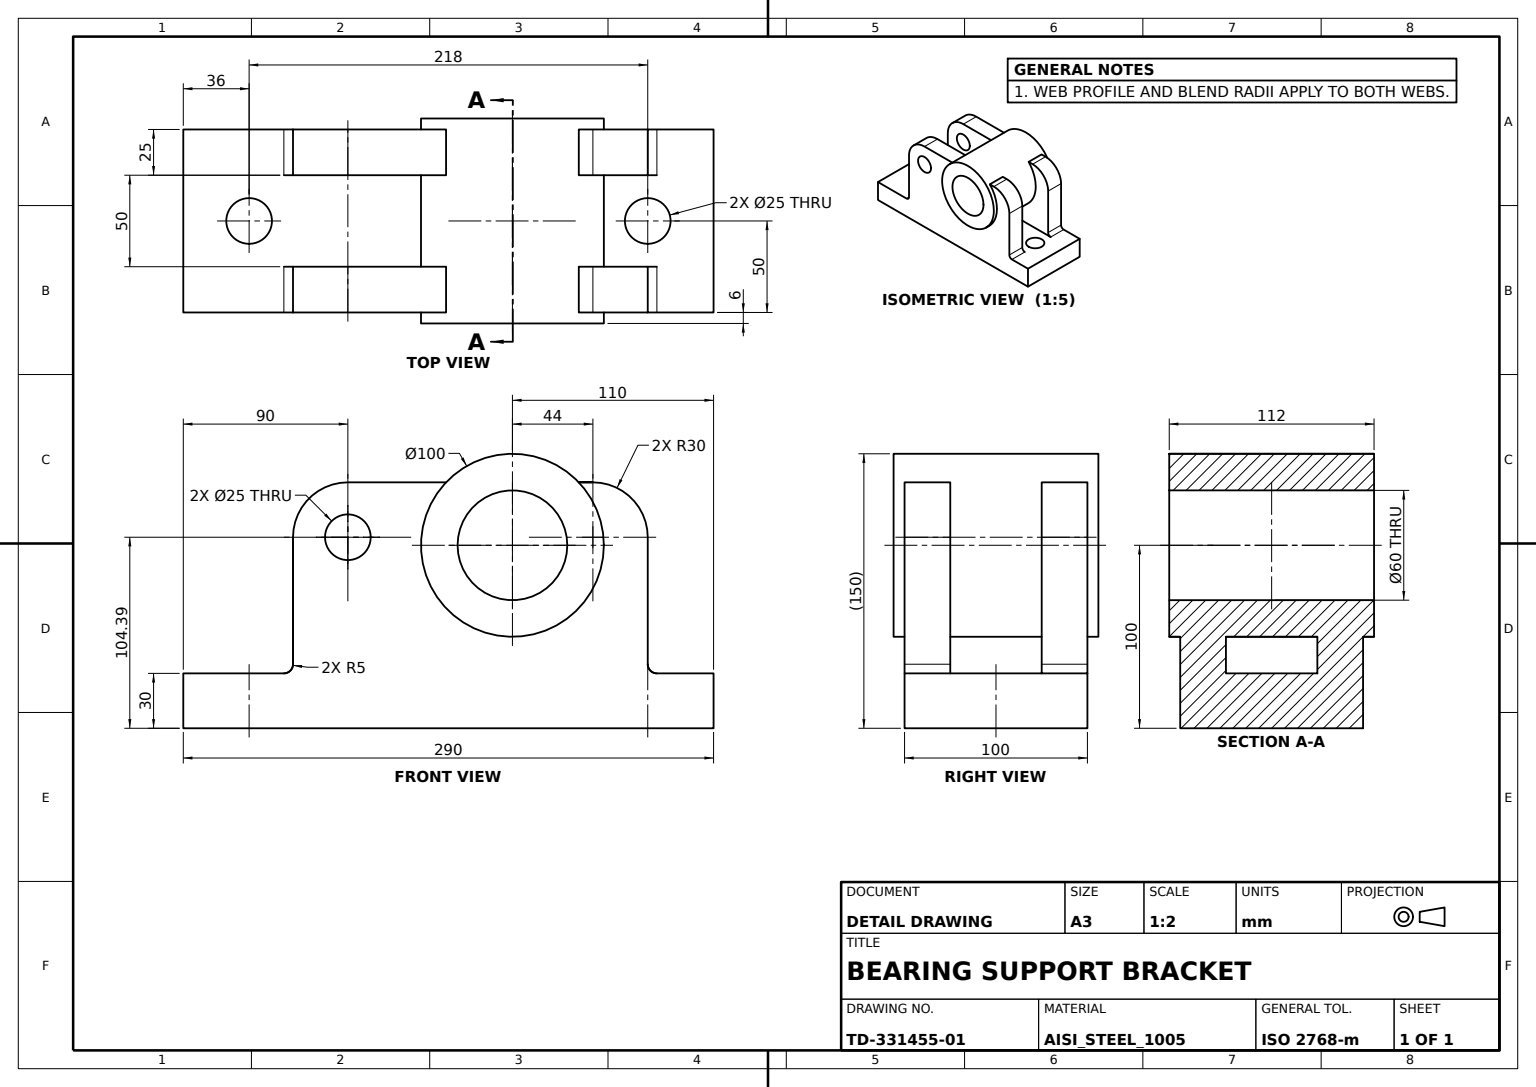
ISO-10303-21;
HEADER;
FILE_DESCRIPTION((''),'2;1');
FILE_NAME('','',(''),(''),'','','');
FILE_SCHEMA(('AUTOMOTIVE_DESIGN'));
ENDSEC;
DATA;
#1=APPLICATION_CONTEXT('');
#2=PRODUCT_CONTEXT('',#1,'mechanical');
#3=PRODUCT('','','',(#2));
#4=PRODUCT_DEFINITION_FORMATION('','',#3);
#5=PRODUCT_DEFINITION_CONTEXT('',#1,'design');
#6=PRODUCT_DEFINITION('','',#4,#5);
#7=PRODUCT_DEFINITION_SHAPE('','',#6);
#8=(LENGTH_UNIT()NAMED_UNIT(*)SI_UNIT(.MILLI.,.METRE.));
#9=(NAMED_UNIT(*)PLANE_ANGLE_UNIT()SI_UNIT($,.RADIAN.));
#10=(NAMED_UNIT(*)SI_UNIT($,.STERADIAN.)SOLID_ANGLE_UNIT());
#11=UNCERTAINTY_MEASURE_WITH_UNIT(LENGTH_MEASURE(0.005),#8,'distance_accuracy_value','');
#12=(GEOMETRIC_REPRESENTATION_CONTEXT(3)GLOBAL_UNCERTAINTY_ASSIGNED_CONTEXT((#11))GLOBAL_UNIT_ASSIGNED_CONTEXT((#8,#9,#10))REPRESENTATION_CONTEXT('',''));
#13=CARTESIAN_POINT('',(-50.,79.,134.393398));
#14=VERTEX_POINT('',#13);
#15=CARTESIAN_POINT('',(-50.,71.291792,134.393398));
#16=VERTEX_POINT('',#15);
#17=DIRECTION('',(0.,1.,0.));
#18=VECTOR('',#17,1000.);
#19=LINE('',#15,#18);
#20=EDGE_CURVE('',#14,#16,#19,.F.);
#21=ORIENTED_EDGE('',*,*,#20,.T.);
#22=CARTESIAN_POINT('',(-25.,71.291792,134.393398));
#23=VERTEX_POINT('',#22);
#24=DIRECTION('',(1.,0.,0.));
#25=VECTOR('',#24,1000.);
#26=LINE('',#15,#25);
#27=EDGE_CURVE('',#16,#23,#26,.T.);
#28=ORIENTED_EDGE('',*,*,#27,.T.);
#29=CARTESIAN_POINT('',(-25.,79.,134.393398));
#30=VERTEX_POINT('',#29);
#31=LINE('',#22,#18);
#32=EDGE_CURVE('',#30,#23,#31,.F.);
#33=ORIENTED_EDGE('',*,*,#32,.F.);
#34=LINE('',#13,#25);
#35=EDGE_CURVE('',#14,#30,#34,.T.);
#36=ORIENTED_EDGE('',*,*,#35,.F.);
#37=EDGE_LOOP('',(#21,#28,#33,#36));
#38=FACE_BOUND('',#37,.T.);
#39=DIRECTION('',(0.,0.,-1.));
#40=DIRECTION('',(-1.,0.,0.));
#41=AXIS2_PLACEMENT_3D('',#15,#39,#40);
#42=PLANE('',#41);
#43=ADVANCED_FACE('',(#38),#42,.F.);
#44=CARTESIAN_POINT('',(25.,-42.5,104.393398));
#45=VERTEX_POINT('',#44);
#46=CARTESIAN_POINT('',(25.,-55.,104.393398));
#47=AXIS2_PLACEMENT_3D('',#46,#24,#17);
#48=CIRCLE('',#47,12.5);
#49=EDGE_CURVE('',#45,#45,#48,.T.);
#50=ORIENTED_EDGE('',*,*,#49,.F.);
#51=EDGE_LOOP('',(#50));
#52=FACE_BOUND('',#51,.T.);
#53=CARTESIAN_POINT('',(50.,-42.5,104.393398));
#54=VERTEX_POINT('',#53);
#55=CARTESIAN_POINT('',(50.,-55.,104.393398));
#56=AXIS2_PLACEMENT_3D('',#55,#24,#17);
#57=CIRCLE('',#56,12.5);
#58=EDGE_CURVE('',#54,#54,#57,.T.);
#59=ORIENTED_EDGE('',*,*,#58,.T.);
#60=EDGE_LOOP('',(#59));
#61=FACE_BOUND('',#60,.T.);
#62=DIRECTION('',(0.,0.,1.));
#63=AXIS2_PLACEMENT_3D('',#55,#40,#62);
#64=CYLINDRICAL_SURFACE('',#63,12.5);
#65=ADVANCED_FACE('',(#52,#61),#64,.F.);
#66=CARTESIAN_POINT('',(50.,-145.,30.));
#67=VERTEX_POINT('',#66);
#68=CARTESIAN_POINT('',(50.,-145.,0.));
#69=VERTEX_POINT('',#68);
#70=VECTOR('',#39,1000.);
#71=LINE('',#66,#70);
#72=EDGE_CURVE('',#67,#69,#71,.T.);
#73=ORIENTED_EDGE('',*,*,#72,.F.);
#74=CARTESIAN_POINT('',(-50.,-145.,30.));
#75=VERTEX_POINT('',#74);
#76=LINE('',#74,#25);
#77=EDGE_CURVE('',#75,#67,#76,.T.);
#78=ORIENTED_EDGE('',*,*,#77,.F.);
#79=CARTESIAN_POINT('',(-50.,-145.,0.));
#80=VERTEX_POINT('',#79);
#81=LINE('',#74,#70);
#82=EDGE_CURVE('',#75,#80,#81,.T.);
#83=ORIENTED_EDGE('',*,*,#82,.T.);
#84=LINE('',#79,#25);
#85=EDGE_CURVE('',#80,#69,#84,.T.);
#86=ORIENTED_EDGE('',*,*,#85,.T.);
#87=EDGE_LOOP('',(#73,#78,#83,#86));
#88=FACE_BOUND('',#87,.T.);
#89=AXIS2_PLACEMENT_3D('',#74,#17,#62);
#90=PLANE('',#89);
#91=ADVANCED_FACE('',(#88),#90,.F.);
#92=CARTESIAN_POINT('',(50.,114.,30.));
#93=VERTEX_POINT('',#92);
#94=CARTESIAN_POINT('',(50.,109.,35.));
#95=VERTEX_POINT('',#94);
#96=CARTESIAN_POINT('',(50.,114.,35.));
#97=DIRECTION('',(0.,-1.,0.));
#98=AXIS2_PLACEMENT_3D('',#96,#40,#97);
#99=CIRCLE('',#98,5.);
#100=EDGE_CURVE('',#93,#95,#99,.T.);
#101=ORIENTED_EDGE('',*,*,#100,.F.);
#102=CARTESIAN_POINT('',(25.,114.,30.));
#103=VERTEX_POINT('',#102);
#104=VECTOR('',#40,1000.);
#105=LINE('',#92,#104);
#106=EDGE_CURVE('',#103,#93,#105,.F.);
#107=ORIENTED_EDGE('',*,*,#106,.F.);
#108=CARTESIAN_POINT('',(25.,109.,35.));
#109=VERTEX_POINT('',#108);
#110=CARTESIAN_POINT('',(25.,114.,35.));
#111=AXIS2_PLACEMENT_3D('',#110,#24,#39);
#112=CIRCLE('',#111,5.);
#113=EDGE_CURVE('',#109,#103,#112,.T.);
#114=ORIENTED_EDGE('',*,*,#113,.F.);
#115=LINE('',#108,#104);
#116=EDGE_CURVE('',#95,#109,#115,.T.);
#117=ORIENTED_EDGE('',*,*,#116,.F.);
#118=EDGE_LOOP('',(#101,#107,#114,#117));
#119=FACE_BOUND('',#118,.T.);
#120=AXIS2_PLACEMENT_3D('',#96,#24,#39);
#121=CYLINDRICAL_SURFACE('',#120,5.);
#122=ADVANCED_FACE('',(#119),#121,.F.);
#123=CARTESIAN_POINT('',(-25.,-90.,30.));
#124=VERTEX_POINT('',#123);
#125=CARTESIAN_POINT('',(-50.,-90.,30.));
#126=VERTEX_POINT('',#125);
#127=LINE('',#125,#25);
#128=EDGE_CURVE('',#124,#126,#127,.F.);
#129=ORIENTED_EDGE('',*,*,#128,.F.);
#130=CARTESIAN_POINT('',(-25.,-85.,35.));
#131=VERTEX_POINT('',#130);
#132=CARTESIAN_POINT('',(-25.,-90.,35.));
#133=AXIS2_PLACEMENT_3D('',#132,#40,#62);
#134=CIRCLE('',#133,5.);
#135=EDGE_CURVE('',#131,#124,#134,.T.);
#136=ORIENTED_EDGE('',*,*,#135,.F.);
#137=CARTESIAN_POINT('',(-50.,-85.,35.));
#138=VERTEX_POINT('',#137);
#139=LINE('',#130,#25);
#140=EDGE_CURVE('',#138,#131,#139,.T.);
#141=ORIENTED_EDGE('',*,*,#140,.F.);
#142=CARTESIAN_POINT('',(-50.,-90.,35.));
#143=AXIS2_PLACEMENT_3D('',#142,#24,#17);
#144=CIRCLE('',#143,5.);
#145=EDGE_CURVE('',#126,#138,#144,.T.);
#146=ORIENTED_EDGE('',*,*,#145,.F.);
#147=EDGE_LOOP('',(#129,#136,#141,#146));
#148=FACE_BOUND('',#147,.T.);
#149=AXIS2_PLACEMENT_3D('',#142,#40,#62);
#150=CYLINDRICAL_SURFACE('',#149,5.);
#151=ADVANCED_FACE('',(#148),#150,.F.);
#152=CARTESIAN_POINT('',(56.,85.,100.));
#153=VERTEX_POINT('',#152);
#154=CARTESIAN_POINT('',(56.,35.,100.));
#155=AXIS2_PLACEMENT_3D('',#154,#24,#17);
#156=CIRCLE('',#155,50.);
#157=EDGE_CURVE('',#153,#153,#156,.T.);
#158=ORIENTED_EDGE('',*,*,#157,.T.);
#159=EDGE_LOOP('',(#158));
#160=FACE_BOUND('',#159,.T.);
#161=CARTESIAN_POINT('',(56.,65.,100.));
#162=VERTEX_POINT('',#161);
#163=CIRCLE('',#155,30.);
#164=EDGE_CURVE('',#162,#162,#163,.F.);
#165=ORIENTED_EDGE('',*,*,#164,.T.);
#166=EDGE_LOOP('',(#165));
#167=FACE_BOUND('',#166,.T.);
#168=AXIS2_PLACEMENT_3D('',#154,#24,#39);
#169=PLANE('',#168);
#170=ADVANCED_FACE('',(#160,#167),#169,.T.);
#171=CARTESIAN_POINT('',(12.5,-109.,30.));
#172=VERTEX_POINT('',#171);
#173=CARTESIAN_POINT('',(0.,-109.,30.));
#174=AXIS2_PLACEMENT_3D('',#173,#62,#24);
#175=CIRCLE('',#174,12.5);
#176=EDGE_CURVE('',#172,#172,#175,.T.);
#177=ORIENTED_EDGE('',*,*,#176,.T.);
#178=EDGE_LOOP('',(#177));
#179=FACE_BOUND('',#178,.T.);
#180=CARTESIAN_POINT('',(12.5,-109.,0.));
#181=VERTEX_POINT('',#180);
#182=CARTESIAN_POINT('',(0.,-109.,0.));
#183=AXIS2_PLACEMENT_3D('',#182,#62,#24);
#184=CIRCLE('',#183,12.5);
#185=EDGE_CURVE('',#181,#181,#184,.T.);
#186=ORIENTED_EDGE('',*,*,#185,.F.);
#187=EDGE_LOOP('',(#186));
#188=FACE_BOUND('',#187,.T.);
#189=AXIS2_PLACEMENT_3D('',#173,#39,#40);
#190=CYLINDRICAL_SURFACE('',#189,12.5);
#191=ADVANCED_FACE('',(#179,#188),#190,.F.);
#192=CARTESIAN_POINT('',(-50.,-42.5,104.393398));
#193=VERTEX_POINT('',#192);
#194=CARTESIAN_POINT('',(-50.,-55.,104.393398));
#195=AXIS2_PLACEMENT_3D('',#194,#24,#17);
#196=CIRCLE('',#195,12.5);
#197=EDGE_CURVE('',#193,#193,#196,.T.);
#198=ORIENTED_EDGE('',*,*,#197,.F.);
#199=EDGE_LOOP('',(#198));
#200=FACE_BOUND('',#199,.T.);
#201=CARTESIAN_POINT('',(-25.,-42.5,104.393398));
#202=VERTEX_POINT('',#201);
#203=CARTESIAN_POINT('',(-25.,-55.,104.393398));
#204=AXIS2_PLACEMENT_3D('',#203,#24,#17);
#205=CIRCLE('',#204,12.5);
#206=EDGE_CURVE('',#202,#202,#205,.T.);
#207=ORIENTED_EDGE('',*,*,#206,.T.);
#208=EDGE_LOOP('',(#207));
#209=FACE_BOUND('',#208,.T.);
#210=AXIS2_PLACEMENT_3D('',#194,#24,#39);
#211=CYLINDRICAL_SURFACE('',#210,12.5);
#212=ADVANCED_FACE('',(#200,#209),#211,.F.);
#213=ORIENTED_EDGE('',*,*,#206,.F.);
#214=EDGE_LOOP('',(#213));
#215=FACE_BOUND('',#214,.T.);
#216=CARTESIAN_POINT('',(-25.,-1.291792,134.393398));
#217=VERTEX_POINT('',#216);
#218=CARTESIAN_POINT('',(-25.,-55.,134.393398));
#219=VERTEX_POINT('',#218);
#220=LINE('',#218,#18);
#221=EDGE_CURVE('',#217,#219,#220,.F.);
#222=ORIENTED_EDGE('',*,*,#221,.T.);
#223=CARTESIAN_POINT('',(-25.,-85.,104.393398));
#224=VERTEX_POINT('',#223);
#225=AXIS2_PLACEMENT_3D('',#203,#40,#17);
#226=CIRCLE('',#225,30.);
#227=EDGE_CURVE('',#219,#224,#226,.F.);
#228=ORIENTED_EDGE('',*,*,#227,.T.);
#229=CARTESIAN_POINT('',(-25.,-85.,30.));
#230=VECTOR('',#62,1000.);
#231=LINE('',#229,#230);
#232=EDGE_CURVE('',#224,#131,#231,.F.);
#233=ORIENTED_EDGE('',*,*,#232,.T.);
#234=ORIENTED_EDGE('',*,*,#135,.T.);
#235=CARTESIAN_POINT('',(-25.,114.,30.));
#236=VERTEX_POINT('',#235);
#237=CARTESIAN_POINT('',(-25.,109.,30.));
#238=VECTOR('',#97,1000.);
#239=LINE('',#237,#238);
#240=EDGE_CURVE('',#124,#236,#239,.F.);
#241=ORIENTED_EDGE('',*,*,#240,.T.);
#242=CARTESIAN_POINT('',(-25.,109.,35.));
#243=VERTEX_POINT('',#242);
#244=CARTESIAN_POINT('',(-25.,114.,35.));
#245=AXIS2_PLACEMENT_3D('',#244,#40,#62);
#246=CIRCLE('',#245,5.);
#247=EDGE_CURVE('',#236,#243,#246,.T.);
#248=ORIENTED_EDGE('',*,*,#247,.T.);
#249=CARTESIAN_POINT('',(-25.,109.,104.393398));
#250=VERTEX_POINT('',#249);
#251=LINE('',#249,#70);
#252=EDGE_CURVE('',#243,#250,#251,.F.);
#253=ORIENTED_EDGE('',*,*,#252,.T.);
#254=CARTESIAN_POINT('',(-25.,79.,104.393398));
#255=AXIS2_PLACEMENT_3D('',#254,#40,#17);
#256=CIRCLE('',#255,30.);
#257=EDGE_CURVE('',#250,#30,#256,.F.);
#258=ORIENTED_EDGE('',*,*,#257,.T.);
#259=ORIENTED_EDGE('',*,*,#32,.T.);
#260=CARTESIAN_POINT('',(-25.,35.,100.));
#261=AXIS2_PLACEMENT_3D('',#260,#24,#17);
#262=CIRCLE('',#261,50.);
#263=EDGE_CURVE('',#23,#217,#262,.F.);
#264=ORIENTED_EDGE('',*,*,#263,.T.);
#265=EDGE_LOOP('',(#222,#228,#233,#234,#241,#248,#253,#258,#259,#264));
#266=FACE_BOUND('',#265,.T.);
#267=AXIS2_PLACEMENT_3D('',#203,#40,#62);
#268=PLANE('',#267);
#269=ADVANCED_FACE('',(#215,#266),#268,.F.);
#270=ORIENTED_EDGE('',*,*,#176,.F.);
#271=EDGE_LOOP('',(#270));
#272=FACE_BOUND('',#271,.T.);
#273=ORIENTED_EDGE('',*,*,#128,.T.);
#274=CARTESIAN_POINT('',(-50.,145.,30.));
#275=LINE('',#274,#238);
#276=EDGE_CURVE('',#126,#75,#275,.T.);
#277=ORIENTED_EDGE('',*,*,#276,.T.);
#278=ORIENTED_EDGE('',*,*,#77,.T.);
#279=CARTESIAN_POINT('',(50.,-90.,30.));
#280=VERTEX_POINT('',#279);
#281=LINE('',#66,#18);
#282=EDGE_CURVE('',#67,#280,#281,.T.);
#283=ORIENTED_EDGE('',*,*,#282,.T.);
#284=CARTESIAN_POINT('',(25.,-90.,30.));
#285=VERTEX_POINT('',#284);
#286=LINE('',#284,#104);
#287=EDGE_CURVE('',#280,#285,#286,.T.);
#288=ORIENTED_EDGE('',*,*,#287,.T.);
#289=CARTESIAN_POINT('',(25.,-85.,30.));
#290=LINE('',#289,#18);
#291=EDGE_CURVE('',#285,#103,#290,.T.);
#292=ORIENTED_EDGE('',*,*,#291,.T.);
#293=ORIENTED_EDGE('',*,*,#106,.T.);
#294=CARTESIAN_POINT('',(50.,145.,30.));
#295=VERTEX_POINT('',#294);
#296=EDGE_CURVE('',#93,#295,#281,.T.);
#297=ORIENTED_EDGE('',*,*,#296,.T.);
#298=VERTEX_POINT('',#274);
#299=LINE('',#294,#104);
#300=EDGE_CURVE('',#295,#298,#299,.T.);
#301=ORIENTED_EDGE('',*,*,#300,.T.);
#302=CARTESIAN_POINT('',(-50.,114.,30.));
#303=VERTEX_POINT('',#302);
#304=EDGE_CURVE('',#298,#303,#275,.T.);
#305=ORIENTED_EDGE('',*,*,#304,.T.);
#306=LINE('',#235,#25);
#307=EDGE_CURVE('',#303,#236,#306,.T.);
#308=ORIENTED_EDGE('',*,*,#307,.T.);
#309=ORIENTED_EDGE('',*,*,#240,.F.);
#310=EDGE_LOOP('',(#273,#277,#278,#283,#288,#292,#293,#297,#301,#305,#308,#309));
#311=FACE_BOUND('',#310,.T.);
#312=CARTESIAN_POINT('',(12.5,109.,30.));
#313=VERTEX_POINT('',#312);
#314=CARTESIAN_POINT('',(0.,109.,30.));
#315=AXIS2_PLACEMENT_3D('',#314,#39,#24);
#316=CIRCLE('',#315,12.5);
#317=EDGE_CURVE('',#313,#313,#316,.T.);
#318=ORIENTED_EDGE('',*,*,#317,.T.);
#319=EDGE_LOOP('',(#318));
#320=FACE_BOUND('',#319,.T.);
#321=AXIS2_PLACEMENT_3D('',#314,#39,#40);
#322=PLANE('',#321);
#323=ADVANCED_FACE('',(#272,#311,#320),#322,.F.);
#324=ORIENTED_EDGE('',*,*,#185,.T.);
#325=EDGE_LOOP('',(#324));
#326=FACE_BOUND('',#325,.T.);
#327=CARTESIAN_POINT('',(50.,145.,0.));
#328=VERTEX_POINT('',#327);
#329=CARTESIAN_POINT('',(-50.,145.,0.));
#330=VERTEX_POINT('',#329);
#331=LINE('',#327,#104);
#332=EDGE_CURVE('',#328,#330,#331,.T.);
#333=ORIENTED_EDGE('',*,*,#332,.F.);
#334=LINE('',#68,#18);
#335=EDGE_CURVE('',#69,#328,#334,.T.);
#336=ORIENTED_EDGE('',*,*,#335,.F.);
#337=ORIENTED_EDGE('',*,*,#85,.F.);
#338=LINE('',#329,#238);
#339=EDGE_CURVE('',#330,#80,#338,.T.);
#340=ORIENTED_EDGE('',*,*,#339,.F.);
#341=EDGE_LOOP('',(#333,#336,#337,#340));
#342=FACE_BOUND('',#341,.T.);
#343=CARTESIAN_POINT('',(12.5,109.,0.));
#344=VERTEX_POINT('',#343);
#345=CARTESIAN_POINT('',(0.,109.,0.));
#346=AXIS2_PLACEMENT_3D('',#345,#39,#24);
#347=CIRCLE('',#346,12.5);
#348=EDGE_CURVE('',#344,#344,#347,.T.);
#349=ORIENTED_EDGE('',*,*,#348,.F.);
#350=EDGE_LOOP('',(#349));
#351=FACE_BOUND('',#350,.T.);
#352=AXIS2_PLACEMENT_3D('',#345,#39,#40);
#353=PLANE('',#352);
#354=ADVANCED_FACE('',(#326,#342,#351),#353,.T.);
#355=ORIENTED_EDGE('',*,*,#164,.F.);
#356=EDGE_LOOP('',(#355));
#357=FACE_BOUND('',#356,.T.);
#358=CARTESIAN_POINT('',(-56.,65.,100.));
#359=VERTEX_POINT('',#358);
#360=CARTESIAN_POINT('',(-56.,35.,100.));
#361=AXIS2_PLACEMENT_3D('',#360,#24,#17);
#362=CIRCLE('',#361,30.);
#363=EDGE_CURVE('',#359,#359,#362,.F.);
#364=ORIENTED_EDGE('',*,*,#363,.T.);
#365=EDGE_LOOP('',(#364));
#366=FACE_BOUND('',#365,.T.);
#367=AXIS2_PLACEMENT_3D('',#360,#24,#39);
#368=CYLINDRICAL_SURFACE('',#367,30.);
#369=ADVANCED_FACE('',(#357,#366),#368,.F.);
#370=ORIENTED_EDGE('',*,*,#257,.F.);
#371=CARTESIAN_POINT('',(-50.,109.,104.393398));
#372=VERTEX_POINT('',#371);
#373=LINE('',#371,#25);
#374=EDGE_CURVE('',#372,#250,#373,.T.);
#375=ORIENTED_EDGE('',*,*,#374,.F.);
#376=CARTESIAN_POINT('',(-50.,79.,104.393398));
#377=AXIS2_PLACEMENT_3D('',#376,#40,#17);
#378=CIRCLE('',#377,30.);
#379=EDGE_CURVE('',#372,#14,#378,.F.);
#380=ORIENTED_EDGE('',*,*,#379,.T.);
#381=ORIENTED_EDGE('',*,*,#35,.T.);
#382=EDGE_LOOP('',(#370,#375,#380,#381));
#383=FACE_BOUND('',#382,.T.);
#384=AXIS2_PLACEMENT_3D('',#376,#24,#39);
#385=CYLINDRICAL_SURFACE('',#384,30.);
#386=ADVANCED_FACE('',(#383),#385,.T.);
#387=LINE('',#274,#70);
#388=EDGE_CURVE('',#298,#330,#387,.T.);
#389=ORIENTED_EDGE('',*,*,#388,.F.);
#390=ORIENTED_EDGE('',*,*,#300,.F.);
#391=LINE('',#294,#70);
#392=EDGE_CURVE('',#295,#328,#391,.T.);
#393=ORIENTED_EDGE('',*,*,#392,.T.);
#394=ORIENTED_EDGE('',*,*,#332,.T.);
#395=EDGE_LOOP('',(#389,#390,#393,#394));
#396=FACE_BOUND('',#395,.T.);
#397=AXIS2_PLACEMENT_3D('',#294,#97,#39);
#398=PLANE('',#397);
#399=ADVANCED_FACE('',(#396),#398,.F.);
#400=CARTESIAN_POINT('',(50.,109.,104.393398));
#401=VERTEX_POINT('',#400);
#402=CARTESIAN_POINT('',(25.,109.,104.393398));
#403=VERTEX_POINT('',#402);
#404=LINE('',#400,#104);
#405=EDGE_CURVE('',#401,#403,#404,.T.);
#406=ORIENTED_EDGE('',*,*,#405,.F.);
#407=CARTESIAN_POINT('',(50.,109.,30.));
#408=LINE('',#407,#230);
#409=EDGE_CURVE('',#95,#401,#408,.T.);
#410=ORIENTED_EDGE('',*,*,#409,.F.);
#411=ORIENTED_EDGE('',*,*,#116,.T.);
#412=CARTESIAN_POINT('',(25.,109.,30.));
#413=LINE('',#412,#230);
#414=EDGE_CURVE('',#109,#403,#413,.T.);
#415=ORIENTED_EDGE('',*,*,#414,.T.);
#416=EDGE_LOOP('',(#406,#410,#411,#415));
#417=FACE_BOUND('',#416,.T.);
#418=AXIS2_PLACEMENT_3D('',#407,#97,#39);
#419=PLANE('',#418);
#420=ADVANCED_FACE('',(#417),#419,.F.);
#421=CARTESIAN_POINT('',(50.,79.,134.393398));
#422=VERTEX_POINT('',#421);
#423=CARTESIAN_POINT('',(25.,79.,134.393398));
#424=VERTEX_POINT('',#423);
#425=LINE('',#421,#104);
#426=EDGE_CURVE('',#422,#424,#425,.T.);
#427=ORIENTED_EDGE('',*,*,#426,.T.);
#428=CARTESIAN_POINT('',(25.,71.291792,134.393398));
#429=VERTEX_POINT('',#428);
#430=LINE('',#423,#238);
#431=EDGE_CURVE('',#424,#429,#430,.T.);
#432=ORIENTED_EDGE('',*,*,#431,.T.);
#433=CARTESIAN_POINT('',(50.,71.291792,134.393398));
#434=VERTEX_POINT('',#433);
#435=LINE('',#433,#104);
#436=EDGE_CURVE('',#434,#429,#435,.T.);
#437=ORIENTED_EDGE('',*,*,#436,.F.);
#438=LINE('',#421,#238);
#439=EDGE_CURVE('',#422,#434,#438,.T.);
#440=ORIENTED_EDGE('',*,*,#439,.F.);
#441=EDGE_LOOP('',(#427,#432,#437,#440));
#442=FACE_BOUND('',#441,.T.);
#443=AXIS2_PLACEMENT_3D('',#421,#39,#40);
#444=PLANE('',#443);
#445=ADVANCED_FACE('',(#442),#444,.F.);
#446=CARTESIAN_POINT('',(50.,-1.291792,134.393398));
#447=VERTEX_POINT('',#446);
#448=CARTESIAN_POINT('',(50.,-55.,134.393398));
#449=VERTEX_POINT('',#448);
#450=LINE('',#446,#238);
#451=EDGE_CURVE('',#447,#449,#450,.T.);
#452=ORIENTED_EDGE('',*,*,#451,.F.);
#453=CARTESIAN_POINT('',(25.,-1.291792,134.393398));
#454=VERTEX_POINT('',#453);
#455=LINE('',#446,#104);
#456=EDGE_CURVE('',#447,#454,#455,.T.);
#457=ORIENTED_EDGE('',*,*,#456,.T.);
#458=CARTESIAN_POINT('',(25.,-55.,134.393398));
#459=VERTEX_POINT('',#458);
#460=LINE('',#453,#238);
#461=EDGE_CURVE('',#454,#459,#460,.T.);
#462=ORIENTED_EDGE('',*,*,#461,.T.);
#463=LINE('',#448,#104);
#464=EDGE_CURVE('',#449,#459,#463,.T.);
#465=ORIENTED_EDGE('',*,*,#464,.F.);
#466=EDGE_LOOP('',(#452,#457,#462,#465));
#467=FACE_BOUND('',#466,.T.);
#468=AXIS2_PLACEMENT_3D('',#446,#39,#40);
#469=PLANE('',#468);
#470=ADVANCED_FACE('',(#467),#469,.F.);
#471=ORIENTED_EDGE('',*,*,#348,.T.);
#472=EDGE_LOOP('',(#471));
#473=FACE_BOUND('',#472,.T.);
#474=ORIENTED_EDGE('',*,*,#317,.F.);
#475=EDGE_LOOP('',(#474));
#476=FACE_BOUND('',#475,.T.);
#477=CYLINDRICAL_SURFACE('',#321,12.5);
#478=ADVANCED_FACE('',(#473,#476),#477,.F.);
#479=CARTESIAN_POINT('',(-50.,-1.291792,134.393398));
#480=VERTEX_POINT('',#479);
#481=CARTESIAN_POINT('',(-50.,-55.,134.393398));
#482=VERTEX_POINT('',#481);
#483=LINE('',#481,#18);
#484=EDGE_CURVE('',#480,#482,#483,.F.);
#485=ORIENTED_EDGE('',*,*,#484,.T.);
#486=LINE('',#481,#25);
#487=EDGE_CURVE('',#482,#219,#486,.T.);
#488=ORIENTED_EDGE('',*,*,#487,.T.);
#489=ORIENTED_EDGE('',*,*,#221,.F.);
#490=LINE('',#479,#25);
#491=EDGE_CURVE('',#480,#217,#490,.T.);
#492=ORIENTED_EDGE('',*,*,#491,.F.);
#493=EDGE_LOOP('',(#485,#488,#489,#492));
#494=FACE_BOUND('',#493,.T.);
#495=AXIS2_PLACEMENT_3D('',#481,#39,#40);
#496=PLANE('',#495);
#497=ADVANCED_FACE('',(#494),#496,.F.);
#498=ORIENTED_EDGE('',*,*,#491,.T.);
#499=ORIENTED_EDGE('',*,*,#263,.F.);
#500=ORIENTED_EDGE('',*,*,#27,.F.);
#501=CARTESIAN_POINT('',(-50.,35.,100.));
#502=AXIS2_PLACEMENT_3D('',#501,#24,#17);
#503=CIRCLE('',#502,50.);
#504=EDGE_CURVE('',#16,#480,#503,.F.);
#505=ORIENTED_EDGE('',*,*,#504,.T.);
#506=EDGE_LOOP('',(#498,#499,#500,#505));
#507=FACE_BOUND('',#506,.T.);
#508=ORIENTED_EDGE('',*,*,#456,.F.);
#509=CARTESIAN_POINT('',(50.,35.,100.));
#510=AXIS2_PLACEMENT_3D('',#509,#40,#17);
#511=CIRCLE('',#510,50.);
#512=EDGE_CURVE('',#434,#447,#511,.T.);
#513=ORIENTED_EDGE('',*,*,#512,.F.);
#514=ORIENTED_EDGE('',*,*,#436,.T.);
#515=CARTESIAN_POINT('',(25.,35.,100.));
#516=AXIS2_PLACEMENT_3D('',#515,#40,#17);
#517=CIRCLE('',#516,50.);
#518=EDGE_CURVE('',#429,#454,#517,.T.);
#519=ORIENTED_EDGE('',*,*,#518,.T.);
#520=EDGE_LOOP('',(#508,#513,#514,#519));
#521=FACE_BOUND('',#520,.T.);
#522=CARTESIAN_POINT('',(-56.,85.,100.));
#523=VERTEX_POINT('',#522);
#524=CIRCLE('',#361,50.);
#525=EDGE_CURVE('',#523,#523,#524,.T.);
#526=ORIENTED_EDGE('',*,*,#525,.T.);
#527=EDGE_LOOP('',(#526));
#528=FACE_BOUND('',#527,.T.);
#529=ORIENTED_EDGE('',*,*,#157,.F.);
#530=EDGE_LOOP('',(#529));
#531=FACE_BOUND('',#530,.T.);
#532=CYLINDRICAL_SURFACE('',#367,50.);
#533=ADVANCED_FACE('',(#507,#521,#528,#531),#532,.T.);
#534=ORIENTED_EDGE('',*,*,#82,.F.);
#535=ORIENTED_EDGE('',*,*,#276,.F.);
#536=ORIENTED_EDGE('',*,*,#145,.T.);
#537=CARTESIAN_POINT('',(-50.,-85.,104.393398));
#538=VERTEX_POINT('',#537);
#539=CARTESIAN_POINT('',(-50.,-85.,30.));
#540=LINE('',#539,#230);
#541=EDGE_CURVE('',#538,#138,#540,.F.);
#542=ORIENTED_EDGE('',*,*,#541,.F.);
#543=AXIS2_PLACEMENT_3D('',#194,#40,#17);
#544=CIRCLE('',#543,30.);
#545=EDGE_CURVE('',#482,#538,#544,.F.);
#546=ORIENTED_EDGE('',*,*,#545,.F.);
#547=ORIENTED_EDGE('',*,*,#484,.F.);
#548=ORIENTED_EDGE('',*,*,#504,.F.);
#549=ORIENTED_EDGE('',*,*,#20,.F.);
#550=ORIENTED_EDGE('',*,*,#379,.F.);
#551=CARTESIAN_POINT('',(-50.,109.,35.));
#552=VERTEX_POINT('',#551);
#553=LINE('',#371,#70);
#554=EDGE_CURVE('',#552,#372,#553,.F.);
#555=ORIENTED_EDGE('',*,*,#554,.F.);
#556=CARTESIAN_POINT('',(-50.,114.,35.));
#557=AXIS2_PLACEMENT_3D('',#556,#24,#17);
#558=CIRCLE('',#557,5.);
#559=EDGE_CURVE('',#552,#303,#558,.T.);
#560=ORIENTED_EDGE('',*,*,#559,.T.);
#561=ORIENTED_EDGE('',*,*,#304,.F.);
#562=ORIENTED_EDGE('',*,*,#388,.T.);
#563=ORIENTED_EDGE('',*,*,#339,.T.);
#564=EDGE_LOOP('',(#534,#535,#536,#542,#546,#547,#548,#549,#550,#555,#560,#561,#562,#563));
#565=FACE_BOUND('',#564,.T.);
#566=ORIENTED_EDGE('',*,*,#197,.T.);
#567=EDGE_LOOP('',(#566));
#568=FACE_BOUND('',#567,.T.);
#569=AXIS2_PLACEMENT_3D('',#274,#24,#17);
#570=PLANE('',#569);
#571=ADVANCED_FACE('',(#565,#568),#570,.F.);
#572=ORIENTED_EDGE('',*,*,#307,.F.);
#573=ORIENTED_EDGE('',*,*,#559,.F.);
#574=LINE('',#551,#25);
#575=EDGE_CURVE('',#243,#552,#574,.F.);
#576=ORIENTED_EDGE('',*,*,#575,.F.);
#577=ORIENTED_EDGE('',*,*,#247,.F.);
#578=EDGE_LOOP('',(#572,#573,#576,#577));
#579=FACE_BOUND('',#578,.T.);
#580=CARTESIAN_POINT('',(0.,114.,35.));
#581=AXIS2_PLACEMENT_3D('',#580,#40,#62);
#582=CYLINDRICAL_SURFACE('',#581,5.);
#583=ADVANCED_FACE('',(#579),#582,.F.);
#584=CARTESIAN_POINT('',(50.,-85.,104.393398));
#585=VERTEX_POINT('',#584);
#586=CARTESIAN_POINT('',(25.,-85.,104.393398));
#587=VERTEX_POINT('',#586);
#588=LINE('',#584,#104);
#589=EDGE_CURVE('',#585,#587,#588,.T.);
#590=ORIENTED_EDGE('',*,*,#589,.T.);
#591=CARTESIAN_POINT('',(25.,-85.,35.));
#592=VERTEX_POINT('',#591);
#593=LINE('',#586,#70);
#594=EDGE_CURVE('',#587,#592,#593,.T.);
#595=ORIENTED_EDGE('',*,*,#594,.T.);
#596=CARTESIAN_POINT('',(50.,-85.,35.));
#597=VERTEX_POINT('',#596);
#598=LINE('',#596,#104);
#599=EDGE_CURVE('',#592,#597,#598,.F.);
#600=ORIENTED_EDGE('',*,*,#599,.T.);
#601=LINE('',#584,#70);
#602=EDGE_CURVE('',#585,#597,#601,.T.);
#603=ORIENTED_EDGE('',*,*,#602,.F.);
#604=EDGE_LOOP('',(#590,#595,#600,#603));
#605=FACE_BOUND('',#604,.T.);
#606=AXIS2_PLACEMENT_3D('',#584,#17,#62);
#607=PLANE('',#606);
#608=ADVANCED_FACE('',(#605),#607,.F.);
#609=ORIENTED_EDGE('',*,*,#461,.F.);
#610=ORIENTED_EDGE('',*,*,#518,.F.);
#611=ORIENTED_EDGE('',*,*,#431,.F.);
#612=CARTESIAN_POINT('',(25.,79.,104.393398));
#613=AXIS2_PLACEMENT_3D('',#612,#24,#17);
#614=CIRCLE('',#613,30.);
#615=EDGE_CURVE('',#403,#424,#614,.T.);
#616=ORIENTED_EDGE('',*,*,#615,.F.);
#617=ORIENTED_EDGE('',*,*,#414,.F.);
#618=ORIENTED_EDGE('',*,*,#113,.T.);
#619=ORIENTED_EDGE('',*,*,#291,.F.);
#620=CARTESIAN_POINT('',(25.,-90.,35.));
#621=AXIS2_PLACEMENT_3D('',#620,#24,#39);
#622=CIRCLE('',#621,5.);
#623=EDGE_CURVE('',#285,#592,#622,.T.);
#624=ORIENTED_EDGE('',*,*,#623,.T.);
#625=ORIENTED_EDGE('',*,*,#594,.F.);
#626=CIRCLE('',#47,30.);
#627=EDGE_CURVE('',#459,#587,#626,.T.);
#628=ORIENTED_EDGE('',*,*,#627,.F.);
#629=EDGE_LOOP('',(#609,#610,#611,#616,#617,#618,#619,#624,#625,#628));
#630=FACE_BOUND('',#629,.T.);
#631=ORIENTED_EDGE('',*,*,#49,.T.);
#632=EDGE_LOOP('',(#631));
#633=FACE_BOUND('',#632,.T.);
#634=AXIS2_PLACEMENT_3D('',#612,#24,#39);
#635=PLANE('',#634);
#636=ADVANCED_FACE('',(#630,#633),#635,.F.);
#637=ORIENTED_EDGE('',*,*,#487,.F.);
#638=ORIENTED_EDGE('',*,*,#545,.T.);
#639=LINE('',#537,#25);
#640=EDGE_CURVE('',#538,#224,#639,.T.);
#641=ORIENTED_EDGE('',*,*,#640,.T.);
#642=ORIENTED_EDGE('',*,*,#227,.F.);
#643=EDGE_LOOP('',(#637,#638,#641,#642));
#644=FACE_BOUND('',#643,.T.);
#645=CYLINDRICAL_SURFACE('',#210,30.);
#646=ADVANCED_FACE('',(#644),#645,.T.);
#647=ORIENTED_EDGE('',*,*,#464,.T.);
#648=ORIENTED_EDGE('',*,*,#627,.T.);
#649=ORIENTED_EDGE('',*,*,#589,.F.);
#650=CIRCLE('',#56,30.);
#651=EDGE_CURVE('',#449,#585,#650,.T.);
#652=ORIENTED_EDGE('',*,*,#651,.F.);
#653=EDGE_LOOP('',(#647,#648,#649,#652));
#654=FACE_BOUND('',#653,.T.);
#655=CYLINDRICAL_SURFACE('',#63,30.);
#656=ADVANCED_FACE('',(#654),#655,.T.);
#657=ORIENTED_EDGE('',*,*,#363,.F.);
#658=EDGE_LOOP('',(#657));
#659=FACE_BOUND('',#658,.T.);
#660=ORIENTED_EDGE('',*,*,#525,.F.);
#661=EDGE_LOOP('',(#660));
#662=FACE_BOUND('',#661,.T.);
#663=PLANE('',#367);
#664=ADVANCED_FACE('',(#659,#662),#663,.F.);
#665=ORIENTED_EDGE('',*,*,#426,.F.);
#666=CARTESIAN_POINT('',(50.,79.,104.393398));
#667=AXIS2_PLACEMENT_3D('',#666,#24,#17);
#668=CIRCLE('',#667,30.);
#669=EDGE_CURVE('',#401,#422,#668,.T.);
#670=ORIENTED_EDGE('',*,*,#669,.F.);
#671=ORIENTED_EDGE('',*,*,#405,.T.);
#672=ORIENTED_EDGE('',*,*,#615,.T.);
#673=EDGE_LOOP('',(#665,#670,#671,#672));
#674=FACE_BOUND('',#673,.T.);
#675=AXIS2_PLACEMENT_3D('',#666,#40,#62);
#676=CYLINDRICAL_SURFACE('',#675,30.);
#677=ADVANCED_FACE('',(#674),#676,.T.);
#678=ORIENTED_EDGE('',*,*,#554,.T.);
#679=ORIENTED_EDGE('',*,*,#374,.T.);
#680=ORIENTED_EDGE('',*,*,#252,.F.);
#681=ORIENTED_EDGE('',*,*,#575,.T.);
#682=EDGE_LOOP('',(#678,#679,#680,#681));
#683=FACE_BOUND('',#682,.T.);
#684=AXIS2_PLACEMENT_3D('',#371,#97,#39);
#685=PLANE('',#684);
#686=ADVANCED_FACE('',(#683),#685,.F.);
#687=ORIENTED_EDGE('',*,*,#541,.T.);
#688=ORIENTED_EDGE('',*,*,#140,.T.);
#689=ORIENTED_EDGE('',*,*,#232,.F.);
#690=ORIENTED_EDGE('',*,*,#640,.F.);
#691=EDGE_LOOP('',(#687,#688,#689,#690));
#692=FACE_BOUND('',#691,.T.);
#693=AXIS2_PLACEMENT_3D('',#539,#17,#62);
#694=PLANE('',#693);
#695=ADVANCED_FACE('',(#692),#694,.F.);
#696=CARTESIAN_POINT('',(50.,-90.,35.));
#697=AXIS2_PLACEMENT_3D('',#696,#40,#97);
#698=CIRCLE('',#697,5.);
#699=EDGE_CURVE('',#597,#280,#698,.T.);
#700=ORIENTED_EDGE('',*,*,#699,.F.);
#701=ORIENTED_EDGE('',*,*,#599,.F.);
#702=ORIENTED_EDGE('',*,*,#623,.F.);
#703=ORIENTED_EDGE('',*,*,#287,.F.);
#704=EDGE_LOOP('',(#700,#701,#702,#703));
#705=FACE_BOUND('',#704,.T.);
#706=CARTESIAN_POINT('',(0.,-90.,35.));
#707=AXIS2_PLACEMENT_3D('',#706,#24,#39);
#708=CYLINDRICAL_SURFACE('',#707,5.);
#709=ADVANCED_FACE('',(#705),#708,.F.);
#710=ORIENTED_EDGE('',*,*,#512,.T.);
#711=ORIENTED_EDGE('',*,*,#451,.T.);
#712=ORIENTED_EDGE('',*,*,#651,.T.);
#713=ORIENTED_EDGE('',*,*,#602,.T.);
#714=ORIENTED_EDGE('',*,*,#699,.T.);
#715=ORIENTED_EDGE('',*,*,#282,.F.);
#716=ORIENTED_EDGE('',*,*,#72,.T.);
#717=ORIENTED_EDGE('',*,*,#335,.T.);
#718=ORIENTED_EDGE('',*,*,#392,.F.);
#719=ORIENTED_EDGE('',*,*,#296,.F.);
#720=ORIENTED_EDGE('',*,*,#100,.T.);
#721=ORIENTED_EDGE('',*,*,#409,.T.);
#722=ORIENTED_EDGE('',*,*,#669,.T.);
#723=ORIENTED_EDGE('',*,*,#439,.T.);
#724=EDGE_LOOP('',(#710,#711,#712,#713,#714,#715,#716,#717,#718,#719,#720,#721,#722,#723));
#725=FACE_BOUND('',#724,.T.);
#726=ORIENTED_EDGE('',*,*,#58,.F.);
#727=EDGE_LOOP('',(#726));
#728=FACE_BOUND('',#727,.T.);
#729=AXIS2_PLACEMENT_3D('',#66,#40,#97);
#730=PLANE('',#729);
#731=ADVANCED_FACE('',(#725,#728),#730,.F.);
#732=CLOSED_SHELL('',(#43,#65,#91,#122,#151,#170,#191,#212,#269,#323,#354,#369,#386,#399,#420,#445,#470,#478,#497,#533,#571,#583,#608,#636,#646,#656,#664,#677,#686,#695,#709,#731));
#733=MANIFOLD_SOLID_BREP('',#732);
#734=ADVANCED_BREP_SHAPE_REPRESENTATION('',(#733),#12);
#735=SHAPE_DEFINITION_REPRESENTATION(#7,#734);
ENDSEC;
END-ISO-10303-21;
